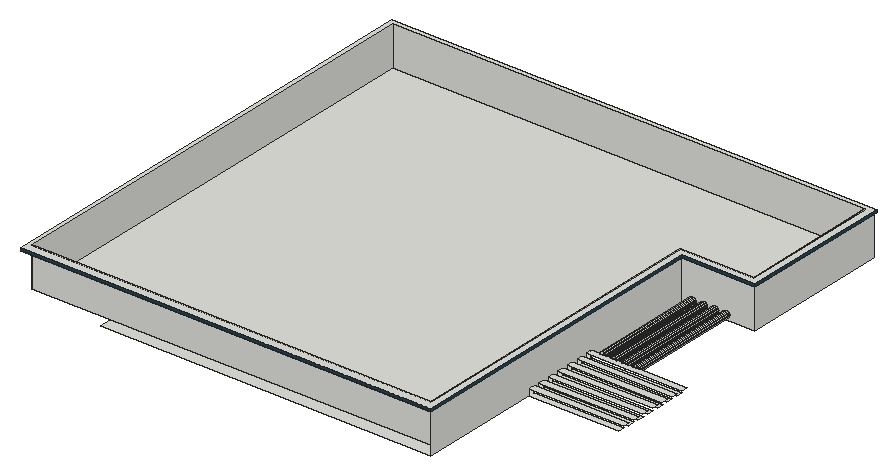
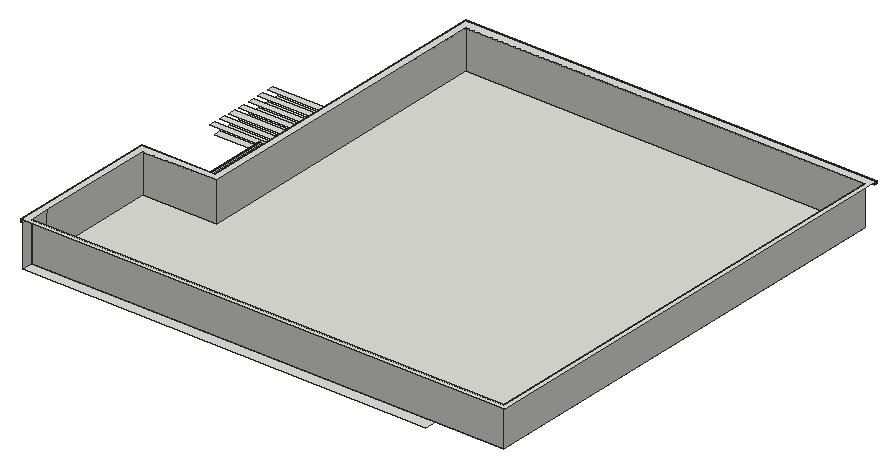
# SketchUp Ruby script. Lengths in millimetres.
U = 1.mm
M = Sketchup.active_model
def pt(a) = Geom::Point3d.new(a.map { |v| v * U })
def face(e, loops, mat)
  f = e.add_face(loops[0].map { |a| pt(a) })
  loops[1..].each { |l| e.add_face(l.map { |a| pt(a) }).erase! }
  f.material = f.back_material = mat if mat
  f
end
# faces: each face lists its corners as indices into pts; further lists are holes
def faces(e, pts, list, mat = nil) = list.each { |f| face(e, (f[0].is_a?(Array) ? f : [f]).map { |l| l.map { |i| pts[i] } }, mat) }
# xy, xz, yz: faces in a plane at the given z, y or x. An outline is a flat list of corners, or four numbers for a rectangle; further outlines are holes
def ring(l) = l.size == 4 ? [[l[0], l[1]], [l[2], l[1]], [l[2], l[3]], [l[0], l[3]]] : l.each_slice(2).to_a
def flat(e, list, mat, &to3) = list.each { |f| face(e, (f[0].is_a?(Array) ? f : [f]).map { |l| ring(l).map { |u, v| to3.(u, v) } }, mat) }
def xy(e, z, list, mat = nil) = flat(e, list, mat) { |x, y| [x, y, z] }
def xz(e, y, list, mat = nil) = flat(e, list, mat) { |x, z| [x, y, z] }
def yz(e, x, list, mat = nil) = flat(e, list, mat) { |y, z| [x, y, z] }
def lines(e, pts, list) = list.each { |a, b| e.add_line(pt(pts[a]), pt(pts[b])) }
# prism: a flat outline (further loops are holes) pulled along v
def prism(e, loops, v, mat = nil)
  f = face(e, loops, mat); d = Geom::Vector3d.new(v.map { |x| x * U })
  f.pushpull(f.normal.samedirection?(d) ? d.length : -d.length)
end
def box(e, o, s, mat = nil) = prism(e, [[o, [o[0] + s[0], o[1], o[2]], [o[0] + s[0], o[1] + s[1], o[2]], [o[0], o[1] + s[1], o[2]]]], [0, 0, s[2]], mat)
def at(x, y, z, deg = 0) = Geom::Transformation.translation(pt([x, y, z])) * Geom::Transformation.rotation(ORIGIN, Z_AXIS, deg.degrees)
def axes(o, x, y, z) = Geom::Transformation.new([*x, 0, *y, 0, *z, 0, *pt(o).to_a, 1])
def part(name) = M.definitions.add(name)
# library, detail: a bought-in or finely detailed component or shape, given as its bounding box
def library(name, o, s) = part(name).tap { |d| box(d.entities, o, s) }
def detail(e, o, s) = box(e.add_group.entities, o, s)
def put(e, d, t, mat = nil) = e.add_instance(d, t).tap { |i| i.material = mat if mat }
def group(e, t, mat = nil) = e.add_group.tap { |g| g.transformation = t; g.material = mat if mat }.entities
root = M.entities
M.materials.add("ThomThom - Jumper2").color = [37, 71, 89]
xy(root,11734.8,[[3733.8,3200.4,3733.8,17602.2,16306.8,17602.2,16306.8,12954,14020.8,12954,14020.8,9449.1,16840.2,9449.1,16840.2,9248.6,14020.8,9248.6,14020.8,9078.8,16840.2,9078.8,16840.2,8875.6,14020.8,8875.6,14020.8,8705.9,16840.2,8705.9,16840.2,8502.7,14020.8,8502.7,14020.8,8332.9,16840.2,8332.9,16840.2,8129.7,14020.8,8129.7,14020.8,7959.9,16840.2,7959.9,16840.2,7756.7,14020.8,7756.7,14020.8,7586.9,16840.2,7586.9,16840.2,7383.7,14020.8,7383.7,14020.8,7213.9,16840.2,7213.9,16840.2,7010.7,14020.8,7010.7,14020.8,3200.4]])
xy(root,11887.2,[[1447.8,3398.8,13868.4,3398.8,13868.4,13106.4,16154.4,13106.4,16154.4,17449.8,1447.8,17449.8]])
xy(root,11938,[[14020.8,7010.7,16992.6,7213.9],[14020.8,7383.7,16992.6,7586.9],[14020.8,7756.7,16992.6,7959.9],[14020.8,8129.7,16992.6,8332.9],[14020.8,8502.7,16992.6,8705.9],
  [14020.8,8875.6,16992.6,9078.8],[14020.8,9248.6,16992.6,9449.1]])
xy(root,13030.2,[[1295.4,3124.2,14097,3200.4],[14020.8,3200.4,14097,12954],[14097,12877.8,16383,12954],[16306.8,12954,16383,17602.2]])
xy(root,13106.4,[[[1295.4,3124.2,14097,3124.2,14097,12877.8,16383,12877.8,16383,17602.2,1295.4,17602.2],[1447.8,3398.8,1447.8,17449.8,16154.4,17449.8,16154.4,13106.4,13868.4,13106.4,13868.4,3398.8]]])
xz(root,3124.2,[[1295.4,13030.2,14097,13106.4]],"ThomThom - Jumper2")
xz(root,3398.8,[[1447.8,11887.2,13868.4,13106.4]])
xz(root,9449.1,[[14377.9,11801.6,14351.7,11805.1,14327.1,11815.3,14306.1,11831.4,14290,11852.4,14279.8,11876.9,14276.3,11903.2,14279.8,11929.5,14283.3,11938,14472.6,11938,14476.1,11929.5,14479.5,11903.2,14476.1,11876.9,14465.9,11852.4,14449.8,11831.4,14428.7,11815.3,14404.2,11805.1],[14732.3,11801.6,14706,11805.1,14681.5,11815.3,14660.4,11831.4,14644.3,11852.4,14634.1,11876.9,14630.7,11903.2,14634.1,11929.5,14637.6,11938,14826.9,11938,14830.4,11929.5,14833.9,11903.2,14830.4,11876.9,14820.2,11852.4,14804.1,11831.4,14783.1,11815.3,14758.6,11805.1],[15080.5,11801.6,15054.2,11805.1,15029.7,11815.3,15008.6,11831.4,14992.5,11852.4,14982.3,11876.9,14978.9,11903.2,14982.3,11929.5,14985.8,11938,15175.1,11938,15178.6,11929.5,15182.1,11903.2,15178.6,11876.9,15168.4,11852.4,15152.3,11831.4,15131.3,11815.3,15106.8,11805.1],[15432.4,11801.6,15406.1,11805.1,15381.6,11815.3,15360.6,11831.4,15344.4,11852.4,15334.3,11876.9,15330.8,11903.2,15334.3,11929.5,15337.8,11938,15527,11938,15530.5,11929.5,15534,11903.2,15530.5,11876.9,15520.4,11852.4,15504.2,11831.4,15483.2,11815.3,15458.7,11805.1],[14283.3,11938,14472.6,11938,14465.9,11954,14449.8,11975.1,14428.7,11991.2,14404.2,12001.4,14377.9,12004.8,14351.7,12001.4,14327.1,11991.2,14306.1,11975.1,14290,11954],
  [14637.6,11938,14826.9,11938,14820.2,11954,14804.1,11975.1,14783.1,11991.2,14758.6,12001.4,14732.3,12004.8,14706,12001.4,14681.5,11991.2,14660.4,11975.1,14644.3,11954],[14985.8,11938,15175.1,11938,15168.4,11954,15152.3,11975.1,15131.3,11991.2,15106.8,12001.4,15080.5,12004.8,15054.2,12001.4,15029.7,11991.2,15008.6,11975.1,14992.5,11954],[15337.8,11938,15527,11938,15520.4,11954,15504.2,11975.1,15483.2,11991.2,15458.7,12001.4,15432.4,12004.8,15406.1,12001.4,15381.6,11991.2,15360.6,11975.1,15344.4,11954]])
xz(root,12877.8,[[14097,13030.2,16383,13106.4]],"ThomThom - Jumper2")
xz(root,12954,[[[14020.8,11734.8,16306.8,13030.2],[14377.9,11801.6,14351.7,11805.1,14327.1,11815.3,14306.1,11831.4,14290,11852.4,14279.8,11876.9,14276.3,11903.2,14279.8,11929.5,14290,11954,14306.1,11975.1,14327.1,11991.2,14351.7,12001.4,14377.9,12004.8,14404.2,12001.4,14428.7,11991.2,14449.8,11975.1,14465.9,11954,14476.1,11929.5,14479.5,11903.2,14476.1,11876.9,14465.9,11852.4,14449.8,11831.4,14428.7,11815.3,14404.2,11805.1],[15080.5,11801.6,15054.2,11805.1,15029.7,11815.3,15008.6,11831.4,14992.5,11852.4,14982.3,11876.9,14978.9,11903.2,14982.3,11929.5,14992.5,11954,15008.6,11975.1,15029.7,11991.2,15054.2,12001.4,15080.5,12004.8,15106.8,12001.4,15131.3,11991.2,15152.3,11975.1,15168.4,11954,15178.6,11929.5,15182.1,11903.2,15178.6,11876.9,15168.4,11852.4,15152.3,11831.4,15131.3,11815.3,15106.8,11805.1],[14732.3,11801.6,14706,11805.1,14681.5,11815.3,14660.4,11831.4,14644.3,11852.4,14634.1,11876.9,14630.7,11903.2,14634.1,11929.5,14644.3,11954,14660.4,11975.1,14681.5,11991.2,14706,12001.4,14732.3,12004.8,14758.6,12001.4,14783.1,11991.2,14804.1,11975.1,14820.2,11954,14830.4,11929.5,14833.9,11903.2,14830.4,11876.9,14820.2,11852.4,14804.1,11831.4,14783.1,11815.3,14758.6,11805.1],[15432.4,11801.6,15406.1,11805.1,15381.6,11815.3,15360.6,11831.4,15344.4,11852.4,15334.3,11876.9,15330.8,11903.2,15334.3,11929.5,15344.4,11954,15360.6,11975.1,15381.6,11991.2,15406.1,12001.4,15432.4,12004.8,15458.7,12001.4,15483.2,11991.2,15504.2,11975.1,15520.4,11954,15530.5,11929.5,15534,11903.2,15530.5,11876.9,15520.4,11852.4,15504.2,11831.4,15483.2,11815.3,15458.7,11805.1]]])
xz(root,13106.4,[[13868.4,11887.2,16154.4,13106.4]])
xz(root,17449.8,[[1447.8,11887.2,16154.4,13106.4]])
yz(root,1447.8,[[3398.8,11887.2,17449.8,13106.4]])
yz(root,13868.4,[[3398.8,11887.2,13106.4,13106.4]])
yz(root,14020.8,[[3200.4,11734.8,7010.7,11734.8,7010.7,11938,7213.9,11938,7213.9,11734.8,7383.7,11734.8,7383.7,11938,7586.9,11938,7586.9,11734.8,7756.7,11734.8,7756.7,11938,7959.9,11938,7959.9,11734.8,8129.7,11734.8,8129.7,11938,8332.9,11938,8332.9,11734.8,8502.7,11734.8,8502.7,11938,8705.9,11938,8705.9,11734.8,8875.6,11734.8,8875.6,11938,9078.8,11938,9078.8,11734.8,9248.6,11734.8,9248.6,11938,9451.8,11938,9451.8,11734.8,12954,11734.8,12954,13030.2,3200.4,13030.2],[9449.1,11734.8,9451.8,11938]])
yz(root,14097,[[3124.2,13030.2,12877.8,13106.4]],"ThomThom - Jumper2")
yz(root,16154.4,[[13106.4,11887.2,16840.2,13106.4],[16840.2,11887.2,17449.8,13106.4]])
yz(root,16306.8,[[12954,11734.8,17602.2,13030.2]])
yz(root,16383,[[12877.8,13030.2,17602.2,13106.4]],"ThomThom - Jumper2")
p = [[14351.7,12954,11805.1],[14377.9,12954,11801.6],[14377.9,9449.1,11801.6],[14351.7,9449.1,11805.1],[14404.2,12954,11805.1],[14404.2,9449.1,11805.1],
  [14706,12954,11805.1],[14732.3,12954,11801.6],[14732.3,9449.1,11801.6],[14706,9449.1,11805.1],[14758.6,12954,11805.1],[14758.6,9449.1,11805.1],
  [15054.2,12954,11805.1],[15080.5,12954,11801.6],[15080.5,9449.1,11801.6],[15054.2,9449.1,11805.1],[15106.8,12954,11805.1],[15106.8,9449.1,11805.1],
  [15406.1,12954,11805.1],[15432.4,12954,11801.6],[15432.4,9449.1,11801.6],[15406.1,9449.1,11805.1],[15458.7,12954,11805.1],[15458.7,9449.1,11805.1],
  [14327.1,12954,11815.3],[14327.1,9449.1,11815.3],[14428.7,12954,11815.3],[14428.7,9449.1,11815.3],[14681.5,12954,11815.3],[14681.5,9449.1,11815.3],
  [14783.1,12954,11815.3],[14783.1,9449.1,11815.3],[15029.7,12954,11815.3],[15029.7,9449.1,11815.3],[15131.3,12954,11815.3],[15131.3,9449.1,11815.3],
  [15381.6,12954,11815.3],[15381.6,9449.1,11815.3],[15483.2,12954,11815.3],[15483.2,9449.1,11815.3],[14306.1,12954,11831.4],[14306.1,9449.1,11831.4],
  [14449.8,12954,11831.4],[14449.8,9449.1,11831.4],[14660.4,12954,11831.4],[14660.4,9449.1,11831.4],[14804.1,12954,11831.4],[14804.1,9449.1,11831.4],
  [15008.6,12954,11831.4],[15008.6,9449.1,11831.4],[15152.3,12954,11831.4],[15152.3,9449.1,11831.4],[15360.6,12954,11831.4],[15360.6,9449.1,11831.4],
  [15504.2,12954,11831.4],[15504.2,9449.1,11831.4],[14290,12954,11852.4],[14290,9449.1,11852.4],[14465.9,12954,11852.4],[14465.9,9449.1,11852.4],
  [14644.3,12954,11852.4],[14644.3,9449.1,11852.4],[14820.2,12954,11852.4],[14820.2,9449.1,11852.4],[14992.5,12954,11852.4],[14992.5,9449.1,11852.4],
  [15168.4,12954,11852.4],[15168.4,9449.1,11852.4],[15344.4,12954,11852.4],[15344.4,9449.1,11852.4],[15520.4,12954,11852.4],[15520.4,9449.1,11852.4],
  [14279.8,12954,11876.9],[14279.8,9449.1,11876.9],[14476.1,12954,11876.9],[14476.1,9449.1,11876.9],[14634.1,12954,11876.9],[14634.1,9449.1,11876.9],
  [14830.4,12954,11876.9],[14830.4,9449.1,11876.9],[14982.3,12954,11876.9],[14982.3,9449.1,11876.9],[15178.6,12954,11876.9],[15178.6,9449.1,11876.9],
  [15334.3,12954,11876.9],[15334.3,9449.1,11876.9],[15530.5,12954,11876.9],[15530.5,9449.1,11876.9],[14276.3,12954,11903.2],[14276.3,9449.1,11903.2],
  [14479.5,12954,11903.2],[14479.5,9449.1,11903.2],[14630.7,12954,11903.2],[14630.7,9449.1,11903.2],[14833.9,12954,11903.2],[14833.9,9449.1,11903.2],
  [14978.9,12954,11903.2],[14978.9,9449.1,11903.2],[15182.1,12954,11903.2],[15182.1,9449.1,11903.2],[15330.8,12954,11903.2],[15330.8,9449.1,11903.2],
  [15534,12954,11903.2],[15534,9449.1,11903.2],[14279.8,12954,11929.5],[14279.8,9449.1,11929.5],[14476.1,12954,11929.5],[14476.1,9449.1,11929.5],
  [14634.1,12954,11929.5],[14634.1,9449.1,11929.5],[14830.4,12954,11929.5],[14830.4,9449.1,11929.5],[14982.3,12954,11929.5],[14982.3,9449.1,11929.5],
  [15178.6,12954,11929.5],[15178.6,9449.1,11929.5],[15334.3,12954,11929.5],[15334.3,9449.1,11929.5],[15530.5,12954,11929.5],[15530.5,9449.1,11929.5],
  [14290,12954,11954],[14283.3,9449.1,11938],[14290,9449.1,11954],[14465.9,12954,11954],[14465.9,9449.1,11954],[14472.6,9449.1,11938],
  [14644.3,12954,11954],[14637.6,9449.1,11938],[14644.3,9449.1,11954],[14820.2,12954,11954],[14820.2,9449.1,11954],[14826.9,9449.1,11938],
  [14992.5,12954,11954],[14985.8,9449.1,11938],[14992.5,9449.1,11954],[15168.4,12954,11954],[15168.4,9449.1,11954],[15175.1,9449.1,11938],
  [15344.4,12954,11954],[15337.8,9449.1,11938],[15344.4,9449.1,11954],[15520.4,12954,11954],[15520.4,9449.1,11954],[15527,9449.1,11938],
  [14306.1,12954,11975.1],[14306.1,9449.1,11975.1],[14449.8,12954,11975.1],[14449.8,9449.1,11975.1],[14660.4,12954,11975.1],[14660.4,9449.1,11975.1],
  [14804.1,12954,11975.1],[14804.1,9449.1,11975.1],[15008.6,12954,11975.1],[15008.6,9449.1,11975.1],[15152.3,12954,11975.1],[15152.3,9449.1,11975.1],
  [15360.6,12954,11975.1],[15360.6,9449.1,11975.1],[15504.2,12954,11975.1],[15504.2,9449.1,11975.1],[14327.1,12954,11991.2],[14327.1,9449.1,11991.2],
  [14428.7,12954,11991.2],[14428.7,9449.1,11991.2],[14681.5,12954,11991.2],[14681.5,9449.1,11991.2],[14783.1,12954,11991.2],[14783.1,9449.1,11991.2],
  [15029.7,12954,11991.2],[15029.7,9449.1,11991.2],[15131.3,12954,11991.2],[15131.3,9449.1,11991.2],[15381.6,12954,11991.2],[15381.6,9449.1,11991.2],
  [15483.2,12954,11991.2],[15483.2,9449.1,11991.2],[14351.7,12954,12001.4],[14351.7,9449.1,12001.4],[14404.2,12954,12001.4],[14404.2,9449.1,12001.4],
  [14706,12954,12001.4],[14706,9449.1,12001.4],[14758.6,12954,12001.4],[14758.6,9449.1,12001.4],[15054.2,12954,12001.4],[15054.2,9449.1,12001.4],
  [15106.8,12954,12001.4],[15106.8,9449.1,12001.4],[15406.1,12954,12001.4],[15406.1,9449.1,12001.4],[15458.7,12954,12001.4],[15458.7,9449.1,12001.4],
  [14377.9,12954,12004.8],[14377.9,9449.1,12004.8],[14732.3,12954,12004.8],[14732.3,9449.1,12004.8],[15080.5,12954,12004.8],[15080.5,9449.1,12004.8],
  [15432.4,12954,12004.8],[15432.4,9449.1,12004.8]]
faces(root,p,[[0,1,2,3],[1,4,5,2],[6,7,8,9],[7,10,11,8],[12,13,14,15],[13,16,17,14],[18,19,20,21],[19,22,23,20],
  [24,0,3,25],[4,26,27,5],[28,6,9,29],[10,30,31,11],[32,12,15,33],[16,34,35,17],[36,18,21,37],[22,38,39,23],
  [40,24,25,41],[26,42,43,27],[44,28,29,45],[30,46,47,31],[48,32,33,49],[34,50,51,35],[52,36,37,53],[38,54,55,39],
  [56,40,41,57],[42,58,59,43],[60,44,45,61],[46,62,63,47],[64,48,49,65],[50,66,67,51],[68,52,53,69],[54,70,71,55],
  [72,56,57,73],[58,74,75,59],[76,60,61,77],[62,78,79,63],[80,64,65,81],[66,82,83,67],[84,68,69,85],[70,86,87,71],
  [88,72,73,89],[74,90,91,75],[92,76,77,93],[78,94,95,79],[96,80,81,97],[82,98,99,83],[100,84,85,101],[86,102,103,87],
  [104,88,89,105],[90,106,107,91],[108,92,93,109],[94,110,111,95],[112,96,97,113],[98,114,115,99],[116,100,101,117],[102,118,119,103],
  [120,104,105,121,122],[106,123,124,125,107],[126,108,109,127,128],[110,129,130,131,111],[132,112,113,133,134],[114,135,136,137,115],[138,116,117,139,140],[118,141,142,143,119],
  [144,120,122,145],[123,146,147,124],[148,126,128,149],[129,150,151,130],[152,132,134,153],[135,154,155,136],[156,138,140,157],[141,158,159,142],
  [160,144,145,161],[146,162,163,147],[164,148,149,165],[150,166,167,151],[168,152,153,169],[154,170,171,155],[172,156,157,173],[158,174,175,159],
  [176,160,161,177],[162,178,179,163],[180,164,165,181],[166,182,183,167],[184,168,169,185],[170,186,187,171],[188,172,173,189],[174,190,191,175],
  [192,176,177,193],[178,192,193,179],[194,180,181,195],[182,194,195,183],[196,184,185,197],[186,196,197,187],[198,188,189,199],[190,198,199,191]])
